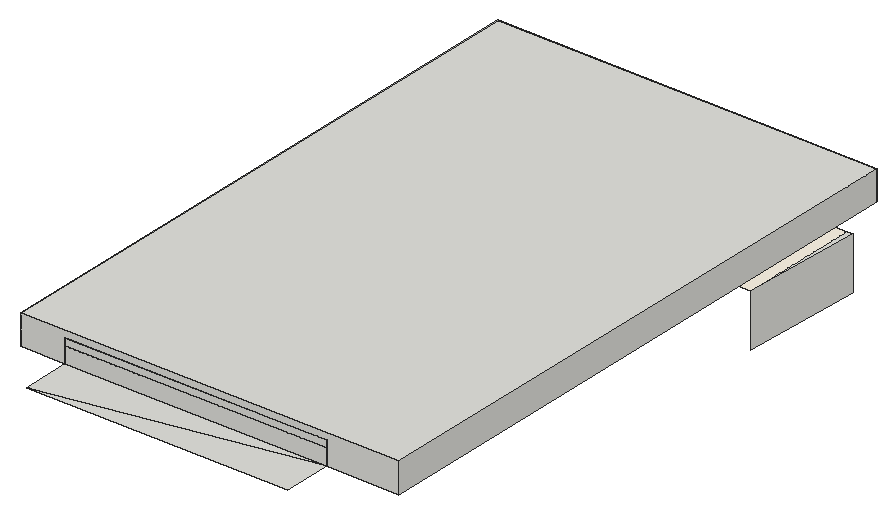
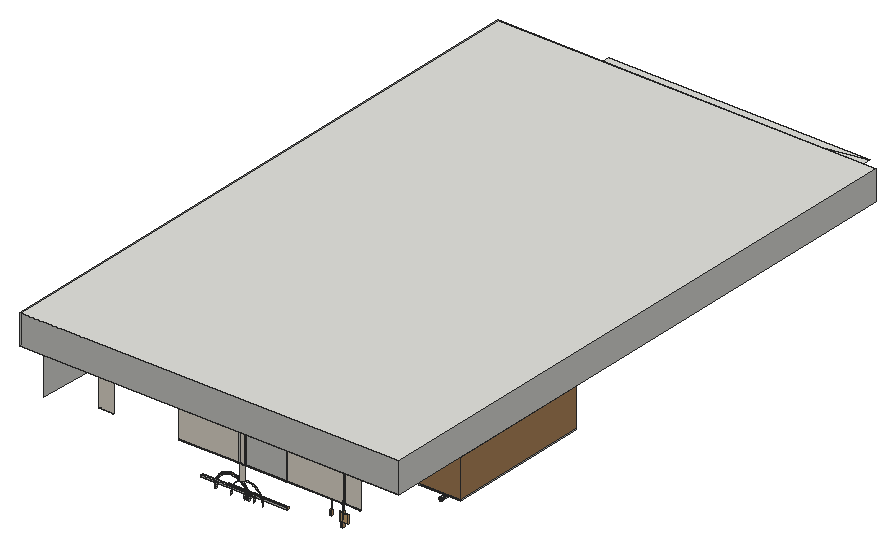
# SketchUp Ruby script. Lengths in inches.
U = 1.inch
M = Sketchup.active_model
def pt(a) = Geom::Point3d.new(a.map { |v| v * U })
def face(e, loops, mat)
  f = e.add_face(loops[0].map { |a| pt(a) })
  loops[1..].each { |l| e.add_face(l.map { |a| pt(a) }).erase! }
  f.material = f.back_material = mat if mat
  f
end
# faces: each face lists its corners as indices into pts; further lists are holes
def faces(e, pts, list, mat = nil) = list.each { |f| face(e, (f[0].is_a?(Array) ? f : [f]).map { |l| l.map { |i| pts[i] } }, mat) }
# xy, xz, yz: faces in a plane at the given z, y or x. An outline is a flat list of corners, or four numbers for a rectangle; further outlines are holes
def ring(l) = l.size == 4 ? [[l[0], l[1]], [l[2], l[1]], [l[2], l[3]], [l[0], l[3]]] : l.each_slice(2).to_a
def flat(e, list, mat, &to3) = list.each { |f| face(e, (f[0].is_a?(Array) ? f : [f]).map { |l| ring(l).map { |u, v| to3.(u, v) } }, mat) }
def xy(e, z, list, mat = nil) = flat(e, list, mat) { |x, y| [x, y, z] }
def xz(e, y, list, mat = nil) = flat(e, list, mat) { |x, z| [x, y, z] }
def yz(e, x, list, mat = nil) = flat(e, list, mat) { |y, z| [x, y, z] }
def lines(e, pts, list) = list.each { |a, b| e.add_line(pt(pts[a]), pt(pts[b])) }
# prism: a flat outline (further loops are holes) pulled along v
def prism(e, loops, v, mat = nil)
  f = face(e, loops, mat); d = Geom::Vector3d.new(v.map { |x| x * U })
  f.pushpull(f.normal.samedirection?(d) ? d.length : -d.length)
end
def box(e, o, s, mat = nil) = prism(e, [[o, [o[0] + s[0], o[1], o[2]], [o[0] + s[0], o[1] + s[1], o[2]], [o[0], o[1] + s[1], o[2]]]], [0, 0, s[2]], mat)
def at(x, y, z, deg = 0) = Geom::Transformation.translation(pt([x, y, z])) * Geom::Transformation.rotation(ORIGIN, Z_AXIS, deg.degrees)
def axes(o, x, y, z) = Geom::Transformation.new([*x, 0, *y, 0, *z, 0, *pt(o).to_a, 1])
def part(name) = M.definitions.add(name)
# library, detail: a bought-in or finely detailed component or shape, given as its bounding box
def library(name, o, s) = part(name).tap { |d| box(d.entities, o, s) }
def detail(e, o, s) = box(e.add_group.entities, o, s)
def put(e, d, t, mat = nil) = e.add_instance(d, t).tap { |i| i.material = mat if mat }
def group(e, t, mat = nil) = e.add_group.tap { |g| g.transformation = t; g.material = mat if mat }.entities
root = M.entities
M.materials.add("Flooring_Parquet_Parallel_H01_120cm").color = [209, 165, 119]
M.materials.add("[0030_OldLace]").color = [253, 245, 230]
M.materials.add("[0129_WhiteSmoke]").color = [245, 245, 245]
M.materials.add("[0134_DimGray]").color = [105, 105, 105]
M.materials.add("[Color A01]").color = [254, 254, 199]
M.materials.add("noyer1").color = [183, 140, 95]
c1 = part("建立群組\#310")
box(c1.entities,[0,0,0],[1.57,1.97,5.51])
c2 = library("Group\#30",[-0.5,-0.5,0],[48.18,1,1.52])
c3 = part("建立群組\#306")
xy(c3.entities,0,[[0.16,0,0.11,0.02,0.07,0.04,0.04,0.08,0.01,0.13,0,0.18,0,0.23,0.02,0.28,0.04,0.32,0.08,0.36,0.13,0.38,0.18,0.39,0.23,0.39,0.28,0.375,0.32,0.35,0.36,0.31,0.38,0.26,0.39,0.21,0.39,0.16,0.375,0.11,0.35,0.07,0.31,0.04,0.26,0.01,0.21,0]])
xy(c3.entities,59.06,[[0.16,0,0.21,0,0.26,0.01,0.31,0.04,0.35,0.07,0.375,0.11,0.39,0.16,0.39,0.21,0.38,0.26,0.36,0.31,0.32,0.35,0.28,0.375,0.23,0.39,0.18,0.39,0.13,0.38,0.08,0.36,0.04,0.32,0.02,0.28,0,0.23,0,0.18,0.01,0.13,0.04,0.08,0.07,0.04,0.11,0.02]])
xz(c3.entities,0,[[0.16,0,0.21,59.06]],"Flooring_Parquet_Parallel_H01_120cm")
xz(c3.entities,0.39,[[0.18,0,0.23,59.06]],"Flooring_Parquet_Parallel_H01_120cm")
yz(c3.entities,0,[[0.18,0,0.23,59.06]],"Flooring_Parquet_Parallel_H01_120cm")
yz(c3.entities,0.39,[[0.16,0,0.21,59.06]],"Flooring_Parquet_Parallel_H01_120cm")
p = [[0.04,0.08,0],[0.07,0.04,0],[0.07,0.04,59.06],[0.04,0.08,59.06],[0.11,0.02,0],[0.11,0.02,59.06],
  [0.16,0,0],[0.16,0,59.06],[0.21,0,0],[0.26,0.01,0],[0.26,0.01,59.06],[0.21,0,59.06],
  [0.31,0.04,0],[0.31,0.04,59.06],[0.35,0.07,0],[0.35,0.07,59.06],[0.01,0.13,0],[0.01,0.13,59.06],
  [0,0.18,0],[0,0.18,59.06],[0.375,0.11,0],[0.375,0.11,59.06],[0.39,0.16,0],[0.39,0.16,59.06],
  [0.02,0.28,0],[0,0.23,0],[0,0.23,59.06],[0.02,0.28,59.06],[0.39,0.21,0],[0.38,0.26,0],
  [0.38,0.26,59.06],[0.39,0.21,59.06],[0.08,0.36,0],[0.04,0.32,0],[0.04,0.32,59.06],[0.08,0.36,59.06],
  [0.32,0.35,0],[0.28,0.375,0],[0.28,0.375,59.06],[0.32,0.35,59.06],[0.36,0.31,0],[0.36,0.31,59.06],
  [0.13,0.38,0],[0.13,0.38,59.06],[0.18,0.39,0],[0.18,0.39,59.06],[0.23,0.39,0],[0.23,0.39,59.06]]
faces(c3.entities,p,[[0,1,2,3],[1,4,5,2],[4,6,7,5],[8,9,10,11],[9,12,13,10],[12,14,15,13],[16,0,3,17],[18,16,17,19],
  [14,20,21,15],[20,22,23,21],[24,25,26,27],[28,29,30,31],[32,33,34,35],[33,24,27,34],[36,37,38,39],[40,36,39,41],
  [29,40,41,30],[42,32,35,43],[44,42,43,45],[37,46,47,38]],"Flooring_Parquet_Parallel_H01_120cm")
c4 = library("建立群組\#5",[-0.5,-0.5,0],[1.79,16.75,15.75])
c5 = part("建立群組\#302")
xy(c5.entities,0,[[-0.04,0,-0.13,0.03,-0.21,0.08,-0.28,0.15,-0.32,0.24,-0.34,0.33,-0.34,0.43,-0.31,0.52,-0.26,0.6,-0.1875,0.67,-0.1,0.71,-0.01,0.73,0.09,0.73,0.18,0.7,0.26,0.65,0.33,0.58,0.37,0.49,0.39,0.4,0.39,0.3,0.36,0.21,0.31,0.13,0.24,0.07,0.15,0.02,0.06,0]])
xy(c5.entities,110.43,[[-0.04,0,0.06,0,0.15,0.02,0.24,0.07,0.31,0.13,0.36,0.21,0.39,0.3,0.39,0.4,0.37,0.49,0.33,0.58,0.26,0.65,0.18,0.7,0.09,0.73,-0.01,0.73,-0.1,0.71,-0.1875,0.67,-0.26,0.6,-0.31,0.52,-0.34,0.43,-0.34,0.33,-0.32,0.24,-0.28,0.15,-0.21,0.08,-0.13,0.03]])
xz(c5.entities,0,[[-0.04,0,0.06,110.43]],"Flooring_Parquet_Parallel_H01_120cm")
xz(c5.entities,0.73,[[-0.01,0,0.09,110.43]],"Flooring_Parquet_Parallel_H01_120cm")
yz(c5.entities,-0.34,[[0.33,0,0.43,110.43]],"Flooring_Parquet_Parallel_H01_120cm")
yz(c5.entities,0.39,[[0.3,0,0.4,110.43]],"Flooring_Parquet_Parallel_H01_120cm")
p = [[-0.21,0.08,0],[-0.13,0.03,0],[-0.13,0.03,110.43],[-0.21,0.08,110.43],[-0.04,0,0],[-0.04,0,110.43],
  [0.06,0,0],[0.15,0.02,0],[0.15,0.02,110.43],[0.06,0,110.43],[0.24,0.07,0],[0.24,0.07,110.43],
  [-0.28,0.15,0],[-0.28,0.15,110.43],[0.31,0.13,0],[0.31,0.13,110.43],[0.36,0.21,0],[0.36,0.21,110.43],
  [-0.32,0.24,0],[-0.32,0.24,110.43],[-0.34,0.33,0],[-0.34,0.33,110.43],[0.39,0.3,0],[0.39,0.3,110.43],
  [-0.31,0.52,0],[-0.34,0.43,0],[-0.34,0.43,110.43],[-0.31,0.52,110.43],[0.39,0.4,0],[0.37,0.49,0],
  [0.37,0.49,110.43],[0.39,0.4,110.43],[-0.26,0.6,0],[-0.26,0.6,110.43],[0.33,0.58,0],[0.33,0.58,110.43],
  [-0.1875,0.67,0],[-0.1875,0.67,110.43],[0.26,0.65,0],[0.18,0.7,0],[0.18,0.7,110.43],[0.26,0.65,110.43],
  [-0.1,0.71,0],[-0.1,0.71,110.43],[-0.01,0.73,0],[-0.01,0.73,110.43],[0.09,0.73,0],[0.09,0.73,110.43]]
faces(c5.entities,p,[[0,1,2,3],[1,4,5,2],[6,7,8,9],[7,10,11,8],[12,0,3,13],[10,14,15,11],[14,16,17,15],[18,12,13,19],
  [20,18,19,21],[16,22,23,17],[24,25,26,27],[28,29,30,31],[32,24,27,33],[29,34,35,30],[36,32,33,37],[38,39,40,41],
  [34,38,41,35],[42,36,37,43],[44,42,43,45],[39,46,47,40]],"Flooring_Parquet_Parallel_H01_120cm")
c6 = library("svet",[-50.16,-50.16,-39.78],[101.06,100.94,121.16])
c7 = library("Group\#31",[-0.5,-0.5,-0.1],[133,18.58,0.2])
xy(root,68.71,[[125.18,500.85,126.7,502.17],[99.22,502.17,125.18,503.68],[125.18,502.17,126.7,503.68],[126.7,502.17,146.4,503.68],[146.4,502.17,167.21,503.68],
  [125.18,503.68,126.7,506.41]])
xy(root,70.22,[[125.18,500.85,126.7,502.17],[99.22,502.17,125.18,503.68],[125.18,502.17,126.7,503.68],[126.7,502.17,146.4,503.68],[146.4,502.17,167.21,503.68],
  [125.18,503.68,126.7,506.41]])
xy(root,85.91,[[2.53,335.23,33.46,450.62]],"noyer1")
xy(root,86.91,[[2.53,335.23,33.46,450.62]],"noyer1")
xy(root,93.02,[[35.9,508.85,48.54,508.97],[48.84,508.85,94.41,508.97],[94.71,508.85,127.66,508.97],[127.96,508.85,132.6,508.97],[132.9,508.85,180.6,508.97],
  [232.6,508.85,244.6,509.16]])
xy(root,93.32,[[35.9,508.85,48.54,508.97],[48.84,508.85,94.41,508.97],[94.71,508.85,127.66,508.97],[127.96,508.85,132.6,508.97],[132.9,508.85,180.6,508.97],
  [232.6,508.85,244.6,509.16]])
xy(root,111.375,[[302.125,390.22,302.125,486.22,306.875,486.22]])
xy(root,111.375,[[244.6,390.22,302.125,486.22]],"[0030_OldLace]")
xy(root,116.89,[[2.53,335.23,35.9,450.62]],"noyer1")
xy(root,120,[[35.9,0,244.6,0,244.6,38.875],[35.9,0,244.6,38.875,35.9,38.875],[0,38.875,0,515.625,302.125,515.625,302.125,38.875,244.6,38.875,244.6,510.22,35.9,510.22,35.9,38.875],[35.9,508.85,48.54,510.22],[48.84,508.85,48.84,508.97,48.54,508.97,48.54,510.22,94.41,510.22,94.41,508.85],
  [94.71,508.85,94.71,508.97,94.41,508.97,94.41,510.22,127.66,510.22,127.66,508.85],[127.96,508.85,127.96,508.97,127.66,508.97,127.66,510.22,132.6,510.22,132.6,508.85],[132.9,508.85,132.9,508.97,132.6,508.97,132.6,510.22,180.6,510.22,180.6,508.85],[232.6,508.85,244.6,510.22],[180.6,509.54,189.03,510.22],
  [224.53,509.54,232.6,510.22],[189.03,509.85,190.82,510.22],[191.46,509.85,193.25,510.22],[193.9,509.85,195.69,510.22],[196.34,509.85,198.13,510.22],
  [198.78,509.85,200.57,510.22],[201.21,509.85,203,510.22],[203.53,509.85,205.32,510.22],[205.84,509.85,207.63,510.22],[208.15,509.85,209.94,510.22],
  [210.46,509.85,212.25,510.22],[212.78,509.85,214.57,510.22],[215.09,509.85,216.88,510.22],[217.4,509.85,219.19,510.22],[219.71,509.85,221.5,510.22],
  [222.03,509.85,223.82,510.22]])
xy(root,120,[[[35.9,38.875,35.9,508.85,48.54,508.85,48.54,508.97,48.84,508.97,48.84,508.85,94.41,508.85,94.41,508.97,94.71,508.97,94.71,508.85,127.66,508.85,127.66,508.97,127.96,508.97,127.96,508.85,132.6,508.85,132.6,508.97,132.9,508.97,132.9,508.85,180.6,508.85,180.6,508.22,189.03,508.22,189.03,509.85,190.82,509.85,190.82,510.22,191.46,510.22,191.46,509.85,193.25,509.85,193.25,510.22,193.9,510.22,193.9,509.85,195.69,509.85,195.69,510.22,196.34,510.22,196.34,509.85,198.13,509.85,198.13,510.22,198.78,510.22,198.78,509.85,200.57,509.85,200.57,510.22,201.21,510.22,201.21,509.85,203,509.85,203,510.22,203.53,510.22,203.53,509.85,205.32,509.85,205.32,510.22,205.84,510.22,205.84,509.85,207.63,509.85,207.63,510.22,208.15,510.22,208.15,509.85,209.94,509.85,209.94,510.22,210.46,510.22,210.46,509.85,212.25,509.85,212.25,510.22,212.78,510.22,212.78,509.85,214.57,509.85,214.57,510.22,215.09,510.22,215.09,509.85,216.88,509.85,216.88,510.22,217.4,510.22,217.4,509.85,219.19,509.85,219.19,510.22,219.71,510.22,219.71,509.85,221.5,509.85,221.5,510.22,222.03,510.22,222.03,509.85,223.82,509.85,223.82,510.22,224.53,510.22,224.53,508.22,232.6,508.22,232.6,508.85,244.6,508.85,244.6,38.875],[54.73,294.45,225.77,491.4]]],"[0129_WhiteSmoke]")
xy(root,120,[[180.6,508.22,189.03,509.54],[224.53,508.22,232.6,509.54]],"noyer1")
xy(root,120.6875,[[[54.73,294.45,225.77,491.4],[56.94,296.67,223.56,489.18]]],"[0129_WhiteSmoke]")
xy(root,121.1875,[[[56.94,296.67,223.56,489.18],[59.24,298.96,221.26,486.89]]],"[0129_WhiteSmoke]")
xy(root,121.875,[[[59.24,298.96,221.26,486.89],[61.7,301.42,218.8,484.43]]])
xy(root,123.33,[[44.82,304.69,61.7,469.88]])
xy(root,123.47,[[61.0625,304.69,61.4375,469.88]])
xy(root,123.84,[[61.0625,304.69,61.4375,469.88]])
xy(root,124.09,[[61.0625,304.69,61.4375,469.88]])
xy(root,124.47,[[61.0625,304.69,61.4375,469.88]])
xy(root,124.72,[[61.0625,304.69,61.4375,469.88]])
xy(root,125.09,[[61.0625,304.69,61.4375,469.88]])
xy(root,125.34,[[61.0625,304.69,61.4375,469.88]])
xy(root,125.72,[[61.0625,304.69,61.4375,469.88]])
xy(root,125.97,[[61.0625,304.69,61.4375,469.88]])
xy(root,126.34,[[61.0625,304.69,61.4375,469.88]])
xy(root,126.59,[[61.0625,304.69,61.4375,469.88]])
xy(root,126.97,[[61.0625,304.69,61.4375,469.88]])
xy(root,127.22,[[61.0625,304.69,61.4375,469.88]])
xy(root,127.59,[[61.0625,304.69,61.4375,469.88]])
xy(root,127.84,[[61.0625,304.69,61.4375,469.88]])
xy(root,128.22,[[61.0625,304.69,61.4375,469.88]])
xy(root,128.47,[[61.0625,304.69,61.4375,469.88]])
xy(root,128.84,[[61.0625,304.69,61.4375,469.88]])
xy(root,129.09,[[61.0625,304.69,61.4375,469.88]])
xy(root,129.47,[[61.0625,304.69,61.4375,469.88]])
xy(root,129.66,[[61.0625,304.69,61.4375,469.88]])
xy(root,130.03,[[61.0625,304.69,61.4375,469.88]])
xy(root,130.28,[[61.0625,304.69,61.4375,469.88]])
xy(root,130.66,[[61.0625,304.69,61.4375,469.88]])
xy(root,130.96,[[44.82,304.69,61.7,469.88]])
xy(root,132.5625,[[[61.7,301.42,218.8,484.43],[73.9375,313.66,206.5625,472.1875]],[78.33,318.06,202.17,467.79]],"[0129_WhiteSmoke]")
xy(root,132.5625,[[[73.9375,313.66,206.5625,472.1875],[78.33,318.06,202.17,467.79]]],"[0134_DimGray]")
xy(root,132.9375,[[35.9,38.875,244.6,510.22]])
xy(root,138.875,[[35.9,38.875,244.6,510.22]])
xy(root,143.8125,[[0,38.875,302.125,515.625]])
xz(root,38.875,[[0,120,35.9,120,35.9,138.875,244.6,138.875,244.6,120,302.125,120,302.125,143.8125,0,143.8125],[35.9,120,244.6,132.9375],[35.9,132.9375,244.6,138.875]])
xz(root,294.45,[[54.73,120,225.77,120.6875]])
xz(root,296.67,[[56.94,120.6875,223.56,121.1875]])
xz(root,298.96,[[59.24,121.1875,221.26,121.875]])
xz(root,301.42,[[61.7,121.875,218.8,132.5625]])
xz(root,304.69,[[[44.82,123.33,61.7,130.96],[61.0625,130.28,61.4375,130.66],[61.0625,129.66,61.4375,130.03],[61.0625,129.09,61.4375,129.47],[61.0625,128.47,61.4375,128.84],[61.0625,127.84,61.4375,128.22],[61.0625,127.22,61.4375,127.59],[61.0625,126.59,61.4375,126.97],[61.0625,125.97,61.4375,126.34],[61.0625,125.34,61.4375,125.72],[61.0625,124.72,61.4375,125.09],[61.0625,124.09,61.4375,124.47],[61.0625,123.47,61.4375,123.84]]])
xz(root,335.23,[[2.53,85.91,33.46,86.91],[33.46,85.91,35.9,86.91],[2.53,86.91,35.9,116.89]])
xz(root,450.62,[[2.53,85.91,33.46,86.91],[33.46,85.91,35.9,86.91]])
xz(root,450.62,[[2.53,86.91,35.9,116.89]],"noyer1")
xz(root,469.88,[[[44.82,123.33,61.7,130.96],[61.0625,130.28,61.4375,130.66],[61.0625,129.66,61.4375,130.03],[61.0625,129.09,61.4375,129.47],[61.0625,128.47,61.4375,128.84],[61.0625,127.84,61.4375,128.22],[61.0625,127.22,61.4375,127.59],[61.0625,126.59,61.4375,126.97],[61.0625,125.97,61.4375,126.34],[61.0625,125.34,61.4375,125.72],[61.0625,124.72,61.4375,125.09],[61.0625,124.09,61.4375,124.47],[61.0625,123.47,61.4375,123.84]]])
xz(root,484.43,[[61.7,121.875,218.8,132.5625]],"[0129_WhiteSmoke]")
xz(root,486.89,[[59.24,121.1875,221.26,121.875]],"[0129_WhiteSmoke]")
xz(root,489.18,[[56.94,120.6875,223.56,121.1875]],"[0129_WhiteSmoke]")
xz(root,491.4,[[54.73,120,225.77,120.6875]],"[0129_WhiteSmoke]")
xz(root,500.85,[[125.18,68.71,126.7,70.22]],"noyer1")
xz(root,502.17,[[125.18,68.71,126.7,70.22]])
xz(root,502.17,[[146.4,68.71,167.21,70.22]],"noyer1")
xz(root,503.68,[[99.22,68.71,125.18,70.22],[125.18,68.71,126.7,70.22],[126.7,68.71,146.4,70.22],[146.4,68.71,167.21,70.22]])
xz(root,507.33,[[127.71,73.1,127.86,73.64,128.31,74.77,128.875,75.85,129.55,76.86,130.33,77.8,131.2,78.65,132.15,79.4,133.08,79.99,133.19,80.06,134.35,80.66,135.58,81.125,136.84,81.47,138.14,81.67,139.45,81.74,140.76,81.67,142.05,81.47,143.32,81.125,144.55,80.66,145.71,80.06,146.8125,79.35,147.58,80.4,146.36,81.1875,145.07,81.84,143.72,82.36,142.32,82.74,140.9,82.96,139.45,83.04,138,82.96,136.57,82.74,135.18,82.36,133.83,81.84,132.54,81.1875,132.38,81.08,131.75,80.68,131.34,80.43,130.26,79.6,129.28,78.67,128.39,77.64,127.625,76.52,126.97,75.33,126.45,74.08,126.26,73.4375,127.17,73.32]],"noyer1")
xz(root,508.85,[[94.71,93.32,127.66,120]])
xz(root,508.85,[[132.6,80.26,132.6,93.02,127.96,93.02,127.96,81.67,128.03,81.67,129.32,81.47,130.59,81.125,131.81,80.66],[35.9,93.32,48.54,120],[48.84,93.32,94.41,120],[127.96,93.32,132.6,120],[132.9,93.32,180.6,120],
  [232.6,93.32,244.6,120]],"[0030_OldLace]")
xz(root,508.97,[[35.9,93.02,48.54,93.32],[48.84,93.02,94.41,93.32],[94.71,93.02,127.66,93.32],[127.96,93.02,132.6,93.32],[132.9,93.02,180.6,93.32]])
xz(root,509.16,[[232.6,93.02,244.6,93.32]])
xz(root,510.22,[[35.9,120,244.6,132.9375],[35.9,132.9375,244.6,138.875]])
xz(root,515.625,[[0,120,302.125,143.8125]])
yz(root,0,[[38.875,120,515.625,143.8125]])
yz(root,2.53,[[335.23,85.91,450.62,86.91]])
yz(root,2.53,[[335.23,86.91,450.62,116.89]],"noyer1")
yz(root,33.46,[[335.23,85.91,450.62,86.91]],"noyer1")
yz(root,35.9,[[38.875,120,510.22,132.9375],[38.875,132.9375,510.22,138.875]])
yz(root,44.82,[[304.69,123.33,469.88,130.96]])
yz(root,48.54,[[508.85,93.32,508.97,120]])
yz(root,48.84,[[508.85,93.32,508.97,120]])
yz(root,54.73,[[294.45,120,491.4,120.6875]],"[0129_WhiteSmoke]")
yz(root,56.94,[[296.67,120.6875,489.18,121.1875]])
yz(root,59.24,[[298.96,121.1875,486.89,121.875]])
yz(root,61.0625,[[304.69,123.47,469.88,123.84],[304.69,124.09,469.88,124.47],[304.69,124.72,469.88,125.09],[304.69,125.34,469.88,125.72],[304.69,125.97,469.88,126.34],
  [304.69,126.59,469.88,126.97],[304.69,127.22,469.88,127.59],[304.69,127.84,469.88,128.22],[304.69,128.47,469.88,128.84],[304.69,129.09,469.88,129.47],
  [304.69,129.66,469.88,130.03],[304.69,130.28,469.88,130.66]])
yz(root,61.4375,[[304.69,123.47,469.88,123.84],[304.69,124.09,469.88,124.47],[304.69,124.72,469.88,125.09],[304.69,125.34,469.88,125.72],[304.69,125.97,469.88,126.34],
  [304.69,126.59,469.88,126.97],[304.69,127.22,469.88,127.59],[304.69,127.84,469.88,128.22],[304.69,128.47,469.88,128.84],[304.69,129.09,469.88,129.47],
  [304.69,129.66,469.88,130.03],[304.69,130.28,469.88,130.66]])
yz(root,61.7,[[[301.42,121.875,484.43,132.5625],[304.69,123.33,469.88,130.96]]],"[0129_WhiteSmoke]")
yz(root,94.41,[[508.85,93.32,508.97,120]])
yz(root,94.71,[[508.85,93.32,508.97,120]])
yz(root,99.22,[[502.17,68.71,503.68,70.22]])
yz(root,125.18,[[500.85,68.71,502.17,70.22],[502.17,68.71,503.68,70.22],[503.68,68.71,506.41,70.22]])
yz(root,126.7,[[500.85,68.71,502.17,70.22],[502.17,68.71,503.68,70.22],[503.68,68.71,506.41,70.22]])
yz(root,127.66,[[508.85,93.32,508.97,120]])
yz(root,127.96,[[508.85,93.32,508.97,120]])
yz(root,132.6,[[508.85,93.32,508.97,120]])
yz(root,132.9,[[508.85,93.32,508.97,120]])
yz(root,146.4,[[502.17,68.71,503.68,70.22]])
yz(root,167.21,[[502.17,68.71,503.68,70.22]])
yz(root,218.8,[[301.42,121.875,484.43,132.5625]],"[0129_WhiteSmoke]")
yz(root,221.26,[[298.96,121.1875,486.89,121.875]])
yz(root,223.56,[[296.67,120.6875,489.18,121.1875]])
yz(root,225.77,[[294.45,120,491.4,120.6875]])
yz(root,244.6,[[38.875,120,510.22,132.9375],[38.875,132.9375,510.22,138.875]])
yz(root,302.125,[[38.875,120,515.625,143.8125]])
p = [[122.13,507.33,68.27],[122.54,507.33,67.28],[122.54,506.41,67.28],[122.13,506.41,68.27],[129.68,507.33,67.28],[130.09,507.33,68.27],
  [130.09,506.41,68.27],[129.68,506.41,67.28],[125.7,507.33,69.34],[125.62,508.04,69.21],[125.7,508.04,67.76],[125.78,507.33,67.68],
  [127.26,507.33,67.84],[126.99,508.04,67.9],[126.92,508.04,69.21],[127.18,507.33,69.34],[153.2,508.04,67.76],[153.28,508.04,69.21],
  [153.28,507.33,69.21],[153.2,507.33,67.76],[151.98,508.04,69.21],[151.91,508.04,67.9],[151.91,507.33,67.9],[151.98,507.33,69.21],
  [114.19,508.85,69.21],[114.26,508.85,67.9],[114.26,508.04,67.9],[114.19,508.04,69.21],[139.18,508.85,67.9],[139.25,508.85,69.21],
  [139.25,508.04,69.21],[139.18,508.04,67.9],[121.99,507.33,69.34],[121.99,506.41,69.34],[130.23,507.33,69.34],[130.23,506.41,69.34],
  [125.78,507.33,70.99],[125.7,508.04,70.66],[126.99,508.04,70.52],[127.26,507.33,70.84],[151.91,508.04,70.52],[151.91,507.33,70.52],
  [153.2,508.04,70.66],[153.2,507.33,70.66],[114.26,508.85,70.52],[114.26,508.04,70.52],[139.18,508.85,70.52],[139.18,508.04,70.52],
  [306.875,486.22,111.375],[302.125,390.22,111.375],[302.125,390.22,69.25],[306.875,486.22,69.25],[122.13,507.33,70.4],[122.13,506.41,70.4],
  [130.09,507.33,70.4],[130.09,506.41,70.4],[122.54,507.33,71.4],[122.54,506.41,71.4],[129.68,507.33,71.4],[129.68,506.41,71.4],
  [127.19,508.04,71.82],[127.5,507.33,72.32],[151.7,508.04,71.82],[151.7,507.33,71.82],[114.46,508.85,71.82],[114.46,508.04,71.82],
  [138.97,508.85,71.82],[138.97,508.04,71.82],[126.04,507.33,72.63],[125.92,508.04,72.09],[152.98,508.04,72.09],[152.98,507.33,72.09],
  [123.19,507.33,72.25],[123.19,506.41,72.25],[129.02,507.33,72.25],[129.02,506.41,72.25],[127.53,508.04,73.08],[127.86,507.33,73.64],
  [127.71,507.33,73.1],[151.37,508.04,73.08],[151.37,507.33,73.08],[114.8,508.85,73.08],[114.8,508.04,73.08],[138.63,508.85,73.08],
  [138.63,508.04,73.08],[126.26,507.33,73.4375],[126.3,508.04,73.48],[152.6,508.04,73.48],[152.6,507.33,73.48],[124.05,507.33,72.91],
  [124.05,506.41,72.91],[128.17,507.33,72.91],[128.17,506.41,72.91],[125.04,507.33,73.32],[125.04,506.41,73.32],[127.17,507.33,73.32],
  [127.17,506.41,73.32],[128,508.04,74.31],[128.31,507.33,74.77],[150.9,508.04,74.31],[150.9,507.33,74.31],[115.27,508.85,74.31],
  [115.27,508.04,74.31],[138.16,508.85,74.31],[138.16,508.04,74.31],[126.11,507.33,73.46],[126.11,506.41,73.46],[126.45,507.33,74.08],
  [126.82,508.04,74.83],[152.08,508.04,74.83],[152.08,507.33,74.83],[126.97,507.33,75.33],[128.875,507.33,75.85],[128.6,508.04,75.47],
  [150.3,508.04,75.47],[150.3,507.33,75.47],[115.87,508.85,75.47],[115.87,508.04,75.47],[137.57,508.85,75.47],[137.57,508.04,75.47],
  [127.47,508.04,76.125],[151.43,508.04,76.125],[151.43,507.33,76.125],[127.625,507.33,76.52],[129.3125,508.04,76.57],[129.55,507.33,76.86],
  [149.59,508.04,76.57],[149.59,507.33,76.57],[116.58,508.85,76.57],[116.58,508.04,76.57],[136.85,508.85,76.57],[136.85,508.04,76.57],
  [128.26,508.04,77.34],[150.64,508.04,77.34],[150.64,507.33,77.34],[128.39,507.33,77.64],[130.14,508.04,77.59],[130.33,507.33,77.8],
  [148.76,508.04,77.59],[148.76,507.33,77.59],[117.41,508.85,77.59],[117.41,508.04,77.59],[136.03,508.85,77.59],[136.03,508.04,77.59],
  [129.17,508.04,78.46],[149.73,508.04,78.46],[149.73,507.33,78.46],[129.28,507.33,78.67],[131.07,508.04,78.52],[147.83,508.04,78.52],
  [147.83,507.33,78.52],[118.34,508.85,78.52],[118.34,508.04,78.52],[135.1,508.85,78.52],[135.1,508.04,78.52],[131.2,507.33,78.65],
  [130.26,507.33,79.6],[130.2,508.04,79.49],[132.09,508.04,79.35],[146.8125,508.04,79.35],[146.8125,507.33,79.35],[148.7,508.04,79.49],
  [148.7,507.33,79.49],[119.35,508.85,79.35],[119.35,508.04,79.35],[134.08,508.85,79.35],[134.08,508.04,79.35],[132.15,507.33,79.4],
  [133.08,508.04,79.99],[145.71,508.04,80.06],[145.71,507.33,80.06],[120.45,508.85,80.06],[120.45,508.04,80.06],[132.98,508.85,80.06],
  [132.98,508.04,80.06],[133.08,507.33,79.99],[131.32,508.04,80.4],[131.34,507.33,80.43],[147.58,508.04,80.4],[147.58,507.33,80.4],
  [133.19,508.04,80.06],[133.19,507.33,80.06],[134.35,508.04,80.66],[134.35,507.33,80.66],[144.55,508.04,80.66],[144.55,507.33,80.66],
  [121.625,508.85,80.66],[121.625,508.04,80.66],[131.81,508.85,80.66],[131.81,508.04,80.66],[132.9,508.85,80.1],[132.6,508.85,80.26],
  [131.75,507.33,80.68],[131.75,508.04,80.68],[146.36,508.04,81.1875],[146.36,507.33,81.1875],[17.79,450.62,80.67],[18.11,450.62,80.54],
  [18.11,335.23,80.54],[17.79,335.23,80.67],[18.45,450.62,80.49],[18.45,335.23,80.49],[18.79,450.62,80.54],[18.79,335.23,80.54],
  [19.1,450.62,80.67],[19.1,335.23,80.67],[17.52,450.62,80.875],[17.52,335.23,80.875],[19.375,450.62,80.875],[19.375,335.23,80.875],
  [132.38,507.33,81.08],[132.38,508.04,81.08],[135.58,508.04,81.125],[135.58,507.33,81.125],[143.32,508.04,81.125],[143.32,507.33,81.125],
  [122.85,508.85,81.125],[122.85,508.04,81.125],[130.59,508.04,81.125],[130.59,508.85,81.125],[17.3125,450.62,81.15],[17.3125,335.23,81.15],
  [19.58,450.62,81.15],[19.58,335.23,81.15],[17.18,450.62,81.46],[17.18,335.23,81.46],[19.72,450.62,81.46],[19.72,335.23,81.46],
  [132.54,508.04,81.1875],[132.54,507.33,81.1875],[136.84,508.04,81.47],[136.84,507.33,81.47],[142.05,508.04,81.47],[142.05,507.33,81.47],
  [124.11,508.85,81.47],[124.11,508.04,81.47],[129.32,508.85,81.47],[129.32,508.04,81.47],[133.83,508.04,81.84],[133.83,507.33,81.84],
  [145.07,508.04,81.84],[145.07,507.33,81.84],[17.14,450.62,81.8],[17.14,335.23,81.8],[19.76,450.62,81.8],[19.76,335.23,81.8],
  [138.14,508.04,81.67],[138.14,507.33,81.67],[140.76,508.04,81.67],[140.76,507.33,81.67],[125.41,508.85,81.67],[125.41,508.04,81.67],
  [128.03,508.85,81.67],[128.03,508.04,81.67],[139.45,508.04,81.74],[139.45,507.33,81.74],[126.72,508.85,81.74],[126.72,508.04,81.74],
  [127.66,508.85,81.69],[127.96,508.85,81.67],[17.18,450.62,82.14],[17.18,335.23,82.14],[19.72,450.62,82.14],[19.72,335.23,82.14],
  [135.18,508.04,82.36],[135.18,507.33,82.36],[143.72,508.04,82.36],[143.72,507.33,82.36],[17.3125,450.62,82.46],[17.3125,335.23,82.46],
  [19.58,450.62,82.46],[19.58,335.23,82.46],[136.57,508.04,82.74],[136.57,507.33,82.74],[142.32,508.04,82.74],[142.32,507.33,82.74],
  [17.52,450.62,82.73],[17.52,335.23,82.73],[19.375,450.62,82.73],[19.375,335.23,82.73],[17.79,450.62,82.94],[17.79,335.23,82.94],
  [19.1,450.62,82.94],[19.1,335.23,82.94],[138,508.04,82.96],[138,507.33,82.96],[140.9,508.04,82.96],[140.9,507.33,82.96],
  [18.11,450.62,83.07],[18.11,335.23,83.07],[18.79,450.62,83.07],[18.79,335.23,83.07],[139.45,508.04,83.04],[139.45,507.33,83.04],
  [18.45,450.62,83.12],[18.45,335.23,83.12],[35.9,508.32,118.09],[35.9,451.82,118.09],[35.9,334.03,118.09],[35.9,277.53,118.09],
  [48.54,508.85,93.32],[48.84,508.85,93.32],[94.41,508.85,93.32],[94.71,508.85,93.32],[127.66,508.85,93.32],[127.96,508.85,93.32],
  [132.6,508.85,93.32],[132.9,508.85,93.32],[306.875,390.22,111.375]]
faces(root,p,[[0,1,2,3],[4,5,6,7],[8,9,10,11],[12,13,14,15],[16,17,18,19],[20,21,22,23],[24,25,26,27],[28,29,30,31],
  [32,0,3,33],[5,34,35,6],[36,37,9,8],[15,14,38,39],[40,20,23,41],[17,42,43,18],[44,24,27,45],[29,46,47,30],
  [48,49,50,51],[52,32,33,53],[34,54,55,35],[56,52,53,57],[54,58,59,55],[39,38,60,61],[62,40,41,63],[64,44,45,65],
  [46,66,67,47],[68,69,37,36],[42,70,71,43],[72,56,57,73],[58,74,75,59],[76,77,60],[61,60,78],[77,78,60],
  [79,62,63,80],[81,64,65,82],[66,83,84,67],[68,85,86,69],[70,87,88,71],[89,72,73,90],[74,91,92,75],[93,89,90,94],
  [78,95,96,92,91],[97,98,76],[77,76,98],[99,79,80,100],[101,81,82,102],[83,103,104,84],[105,93,94,106],[85,105,106,96,95],
  [107,86,85],[86,107,108],[87,109,110,88],[111,108,107],[98,97,112],[113,112,97],[114,99,100,115],[116,101,102,117],
  [103,118,119,104],[108,111,120],[109,121,122,110],[123,120,111],[124,125,113],[112,113,125],[126,114,115,127],[128,116,117,129],
  [118,130,131,119],[120,123,132],[121,133,134,122],[135,132,123],[136,137,124],[125,124,137],[138,126,127,139],[140,128,129,141],
  [130,142,143,131],[132,135,144],[133,145,146,134],[147,144,135],[136,148,137],[149,138,139,150],[151,140,141,152],[142,153,154,143],
  [155,137,148],[147,156,144],[157,144,156],[148,158,155],[159,149,150,160],[145,161,162,146],[163,151,152,164],[153,165,166,154],
  [167,155,158],[158,168,167],[169,159,160,170],[171,163,164,172],[173,174,168,166,165],[175,167,168],[176,157,177],[156,177,157],
  [161,178,179,162],[168,180,181,175],[180,182,183,181],[184,169,170,185],[186,171,172,187],[188,189,174,173,190,191],[177,192,176],[193,176,192],
  [178,194,195,179],[196,197,198,199],[197,200,201,198],[200,202,203,201],[202,204,205,203],[206,196,199,207],[204,208,209,205],[192,210,211,193],
  [182,212,213,183],[214,184,185,215],[216,186,187,217],[218,193,189,188,219],[220,206,207,221],[208,222,223,209],[224,220,221,225],[222,226,227,223],
  [228,211,210,229],[212,230,231,213],[232,214,215,233],[234,216,217,235],[219,236,237,218],[238,228,229,239],[194,240,241,195],[242,224,225,243],
  [226,244,245,227],[230,246,247,231],[248,232,233,249],[250,234,235,251],[236,252,253,237],[246,254,255,247],[254,248,249,255],[256,250,251,257],
  [258,256,257,253,252,259],[260,242,243,261],[244,262,263,245],[264,238,239,265],[240,266,267,241],[268,260,261,269],[262,270,271,263],[272,264,265,273],
  [266,274,275,267],[276,268,269,277],[270,278,279,271],[280,276,277,281],[278,282,283,279],[284,272,273,285],[274,286,287,275],[288,280,281,289],
  [282,290,291,283],[292,284,285,293],[286,292,293,287],[294,288,289,295],[290,294,295,291]])
lines(root,p,[[296,297],[298,299],[300,301],[302,303],[304,305],[306,307],[49,308]])
put(root,c1,axes([58.9,497.39,67.65],[0,-0.85,0],[0.85,0,0],[0,0,0.85]),"Flooring_Parquet_Parallel_H01_120cm")
put(root,c2,at(99.22,502.17,68.71))
put(root,c3,axes([59.56,496.8125,72.34],[0,-0.85,0],[0.85,0,0],[0,0,0.85]))
put(root,c4,axes([53.24,499.6875,73.1],[0,-0.4137,0],[0.4137,0,0],[0,0,0.4137]),"[Color A01]")
put(root,c1,axes([65.66,500.3125,74.875],[0,-0.70766,0],[0.70766,0,0],[0,0,0.70766]),"Flooring_Parquet_Parallel_H01_120cm")
put(root,c3,axes([66.21,499.83,78.78],[0,-0.70766,0],[0.70766,0,0],[0,0,0.70766]))
put(root,c1,axes([56.23,499.85,78.91],[0,-0.4137,0],[0.4137,0,0],[0,0,0.4137]),"Flooring_Parquet_Parallel_H01_120cm")
put(root,c5,axes([56.55,499.57,81.19],[0,-0.4137,0],[0.4137,0,0],[0,0,0.4137]))
put(root,c6,axes([138.13,419.5,105.33],[0.3738,0,0],[0,0.3738,0],[0,0,0.3738]))
put(root,c7,axes([206.24,454.02,132.5625],[-1,0,0],[0,1,0],[0,0,-1]))
